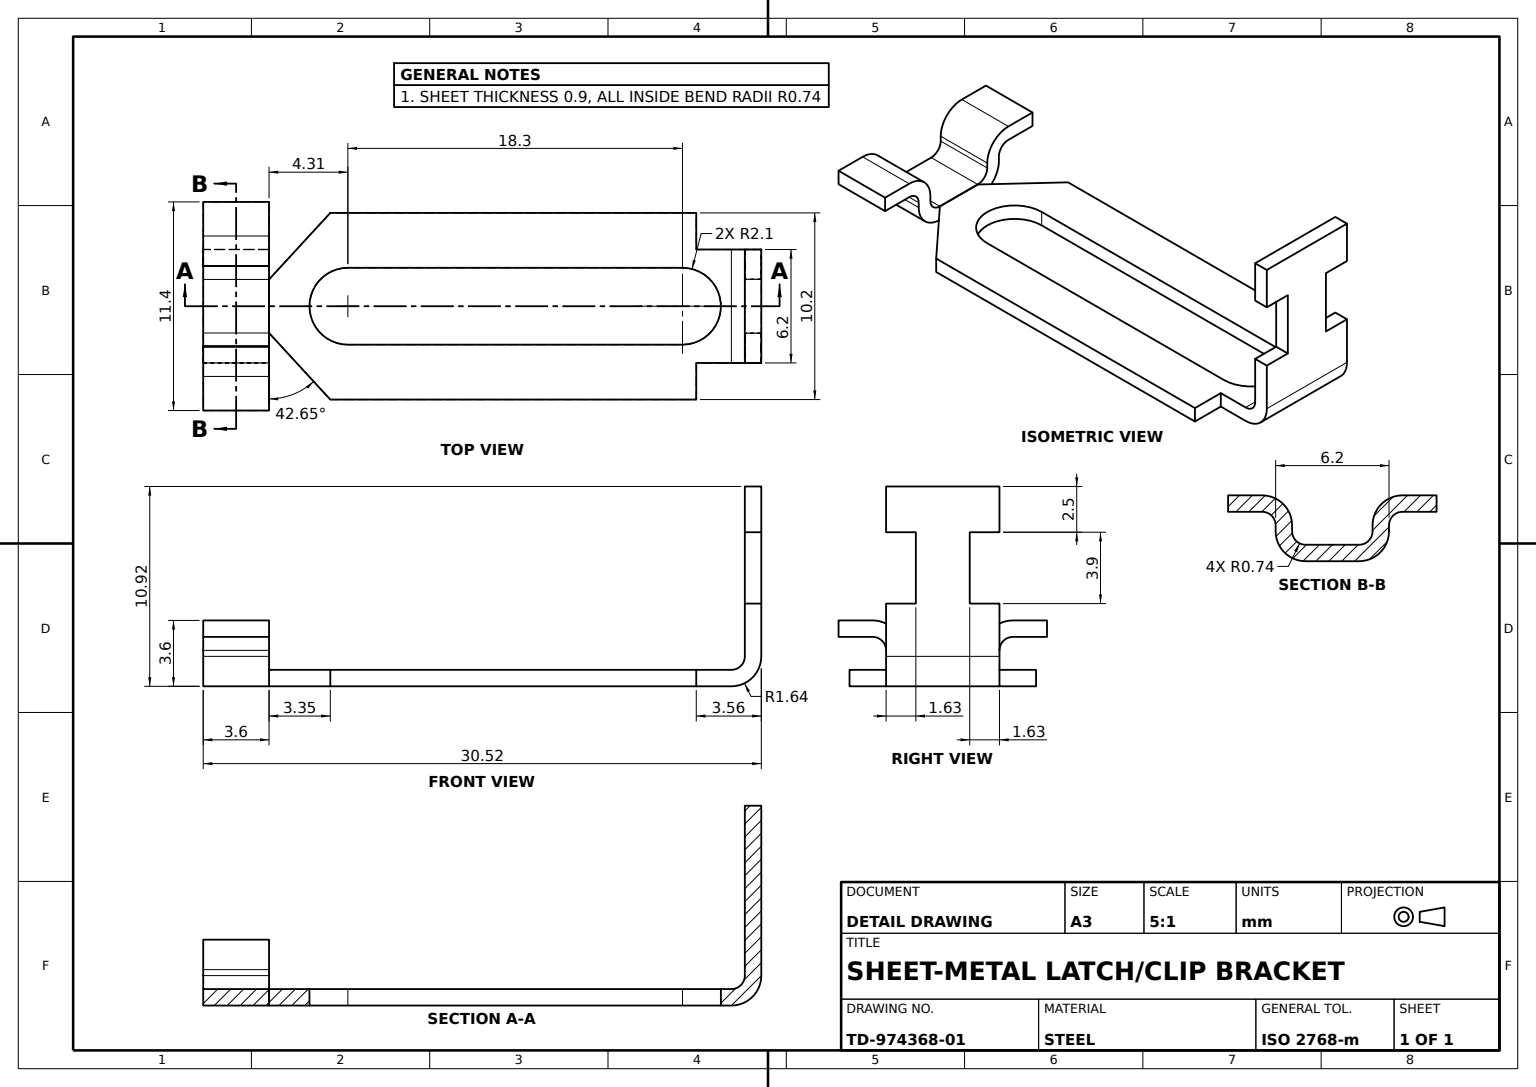
solid
v1 (1.4634,0,13.46)
v2 (1.4634,-0.9,13.46)
e1 v1 v2 LINE
v3 (5.1,-0.9,10.11)
e2 v3 v2 LINE
v4 (5.1,0,10.11)
e3 v3 v4 LINE
e4 v4 v1 LINE
face PLANE(AX(P(1.4634,-3.6,13.46),D(-0.677530464,0,-0.735494712),D(-0.735494712,0,0.677530464))) rev [e1 -e2 e3 e4]
v5 (-3.1,7.52,-12.56)
v6 (-3.1,10.02,-12.56)
e5 v5 v6 LINE
v7 (-3.1,10.02,-13.46)
e6 v7 v6 LINE
v8 (-3.1,7.52,-13.46)
e7 v7 v8 LINE
e8 v8 v5 LINE
face PLANE(AX(P(-3.1,7.958486,-9.86),D(1,0,0),D(0,1,0))) rev [e5 -e6 e7 e8]
v9 (-5.1,0,-9.9034)
v10 (-3.1,0,-9.9034)
e9 v9 v10 LINE
v11 (-3.1,-0.9,-9.9034)
e10 v11 v10 LINE
v12 (-5.1,-0.9,-9.9034)
e11 v12 v11 LINE
e12 v12 v9 LINE
face PLANE(AX(P(-5.1,-3.6,-9.9034),D(0,0,1),D(1,0,0))) rev [e9 -e10 -e11 e12]
v13 (0,0,11.25)
v14 (2.1,0,9.15)
e13 v13 v14 CIRCLE(AX(P(0,0,9.15),D(0,1,0),D(0,0,1)),2.1)
v15 (2.1,-0.9,9.15)
e14 v15 v14 LINE
v16 (0,-0.9,11.25)
e15 v16 v15 CIRCLE(AX(P(0,-0.9,9.15),D(0,1,0),D(0,0,1)),2.1)
e16 v16 v13 LINE
face CYL(AX(P(0,-3.6,9.15),D(0,1,0),D(0,0,1)),2.1) rev [e13 -e14 -e15 e16]
v17 (-3.1,3.62,-12.56)
v18 (-3.1,3.62,-13.46)
e17 v17 v18 LINE
v19 (-1.473197,3.62,-12.56)
e18 v17 v19 LINE
v20 (-1.473197,3.62,-13.46)
e19 v20 v19 LINE
e20 v18 v20 LINE
face PLANE(AX(P(-3.1,3.62,-16.16),D(0,-1,0),D(0,0,-1))) rev [-e17 e18 -e19 -e20]
v21 (3.1,10.02,-12.56)
v22 (3.1,7.52,-12.56)
e21 v21 v22 LINE
e22 v6 v21 LINE
v23 (-1.473197,7.52,-12.56)
e23 v23 v5 LINE
e24 v19 v23 LINE
v24 (-3.1,0.7366,-12.56)
e25 v24 v17 LINE
v25 (3.1,0.7366,-12.56)
e26 v25 v24 LINE
v26 (3.1,3.62,-12.56)
e27 v26 v25 LINE
v27 (1.473197,3.62,-12.56)
e28 v27 v26 LINE
v28 (1.473197,7.52,-12.56)
e29 v28 v27 LINE
e30 v22 v28 LINE
face PLANE(AX(P(0,0,-12.56),D(0,0,1),D(0,-1,0))) [-e21 -e22 -e5 -e23 -e24 -e18 -e25 -e26 -e27 -e28 -e29 -e30]
v29 (-3.1,-0.9,-11.8234)
v30 (3.1,-0.9,-11.8234)
e31 v29 v30 LINE
v31 (-3.1,0.7366,-13.46)
e32 v31 v29 CIRCLE(AX(P(-3.1,0.7366,-11.8234),D(-1,0,0),D(0,0,-1)),1.6366)
v32 (3.1,0.7366,-13.46)
e33 v31 v32 LINE
e34 v30 v32 CIRCLE(AX(P(3.1,0.7366,-11.8234),D(1,0,0),D(0,0,1)),1.6366)
face CYL(AX(P(-5.1,0.7366,-11.8234),D(-1,0,0),D(0,0,-1)),1.6366) [-e31 -e32 e33 -e34]
v33 (-2.1,-0.9,9.15)
v34 (-2.1,0,9.15)
e35 v33 v34 LINE
e36 v34 v13 CIRCLE(AX(P(0,0,9.15),D(0,1,0),D(0,0,1)),2.1)
e37 v33 v16 CIRCLE(AX(P(0,-0.9,9.15),D(0,1,0),D(0,0,1)),2.1)
face CYL(AX(P(0,-3.6,9.15),D(0,1,0),D(0,0,1)),2.1) rev [e35 e36 -e16 -e37]
v35 (-3.1,0,-11.8234)
e38 v10 v35 LINE
v36 (-5.1,0,10.11)
e39 v9 v36 LINE
v37 (-1.4634,0,13.46)
e40 v37 v36 LINE
e41 v37 v1 LINE
v38 (5.1,0,-9.9034)
e42 v4 v38 LINE
v39 (3.1,0,-9.9034)
e43 v39 v38 LINE
v40 (3.1,0,-11.8234)
e44 v40 v39 LINE
e45 v35 v40 LINE
v41 (-2.1,0,-9.15)
e46 v41 v34 LINE
v42 (2.1,0,-9.15)
e47 v42 v41 CIRCLE(AX(P(0,0,-9.15),D(0,1,0),D(0,0,1)),2.1)
e48 v14 v42 LINE
face PLANE(AX(P(0,0,0),D(0,1,0),D(0,0,1))) [-e38 -e9 e39 -e40 e41 -e4 e42 -e43 -e44 -e45] [-e36 -e46 -e47 -e48 -e13]
v43 (-1.473197,7.52,-13.46)
e49 v43 v23 LINE
e50 v20 v43 LINE
face PLANE(AX(P(-1.473197,7.52,-16.16),D(1,0,0),D(0,1,0))) rev [e19 e24 -e49 -e50]
v44 (2.1,-0.9,-9.15)
e51 v15 v44 LINE
v45 (-2.1,-0.9,-9.15)
e52 v44 v45 CIRCLE(AX(P(0,-0.9,-9.15),D(0,1,0),D(0,0,1)),2.1)
e53 v45 v33 LINE
e54 v11 v29 LINE
v46 (3.1,-0.9,-9.9034)
e55 v30 v46 LINE
v47 (5.1,-0.9,-9.9034)
e56 v46 v47 LINE
e57 v3 v47 LINE
v48 (-1.4634,-0.9,13.46)
e58 v48 v2 LINE
v49 (-5.1,-0.9,10.11)
e59 v48 v49 LINE
e60 v12 v49 LINE
face PLANE(AX(P(0,-0.9,0),D(0,1,0),D(0,0,1))) rev [e51 e52 e53 e37 e15] [e54 e31 e55 e56 -e57 e2 -e58 e59 -e60 e11]
e61 v48 v37 LINE
face PLANE(AX(P(-5.1,-0.9,13.46),D(0,0,1),D(1,0,0))) [-e61 e58 -e1 -e41]
v50 (3.1,7.52,-13.46)
e62 v22 v50 LINE
v51 (1.473197,7.52,-13.46)
e63 v51 v28 LINE
e64 v50 v51 LINE
face PLANE(AX(P(3.1,7.52,-16.16),D(0,1,0),D(-1,0,0))) rev [-e62 e30 -e63 -e64]
v52 (3.1,10.02,-13.46)
e65 v52 v21 LINE
e66 v7 v52 LINE
face PLANE(AX(P(5.1,10.02,-13.46),D(0,-1,0),D(0,0,-1))) rev [e6 e22 -e65 -e66]
e67 v44 v42 LINE
e68 v45 v41 LINE
face CYL(AX(P(0,-3.6,-9.15),D(0,1,0),D(0,0,1)),2.1) rev [e67 e47 -e68 -e52]
e69 v47 v38 LINE
face PLANE(AX(P(5.1,-0.9,-13.46),D(1,0,0),D(0,0,-1))) [-e42 -e3 e57 e69]
e70 v49 v36 LINE
face PLANE(AX(P(-1.4634,-3.6,13.46),D(0.677530464,0,-0.735494712),D(-0.735494712,0,-0.677530464))) rev [-e70 -e59 e61 e40]
e71 v46 v39 LINE
face PLANE(AX(P(5.1,-3.6,-9.9034),D(0,0,1),D(1,0,0))) rev [e43 -e69 -e56 e71]
face PLANE(AX(P(2.1,-3.6,9.15),D(1,0,0),D(0,0,-1))) rev [-e67 -e51 e14 e48]
face PLANE(AX(P(-2.1,-3.6,9.15),D(-1,0,0),D(0,0,1))) rev [e46 -e35 -e53 e68]
e72 v50 v52 LINE
v53 (1.473197,3.62,-13.46)
e73 v51 v53 LINE
v54 (3.1,3.62,-13.46)
e74 v53 v54 LINE
e75 v32 v54 LINE
e76 v18 v31 LINE
e77 v43 v8 LINE
face PLANE(AX(P(0,0,-13.46),D(0,0,1),D(0,-1,0))) rev [-e72 e64 e73 e74 -e75 -e33 -e76 e20 e50 e77 -e7 e66]
face PLANE(AX(P(-3.1,7.52,-16.16),D(0,1,0),D(0,0,1))) rev [e49 e23 -e8 -e77]
e78 v54 v26 LINE
e79 v53 v27 LINE
face PLANE(AX(P(3.1,3.62,-16.16),D(0,-1,0),D(0,0,-1))) rev [e28 -e78 -e74 e79]
e80 v40 v25 CIRCLE(AX(P(3.1,0.7366,-11.8234),D(1,0,0),D(0,0,1)),0.7366)
e81 v24 v35 CIRCLE(AX(P(-3.1,0.7366,-11.8234),D(-1,0,0),D(0,0,-1)),0.7366)
face CYL(AX(P(-5.1,0.7366,-11.8234),D(-1,0,0),D(0,0,-1)),0.7366) rev [e45 e80 e26 e81]
face PLANE(AX(P(-3.1,-3.6,-11.8234),D(1,0,0),D(0,0,-1))) rev [e38 -e81 e25 e17 e76 e32 -e54 e10]
face PLANE(AX(P(3.1,7.958486,-9.86),D(-1,0,0),D(0,-1,0))) rev [e62 e72 e65 e21]
face PLANE(AX(P(1.473197,7.52,-16.16),D(-1,0,0),D(0,-1,0))) rev [e63 e29 -e79 -e73]
face PLANE(AX(P(-5.1,-0.9,-13.46),D(-1,0,0),D(0,0,1))) [e70 -e39 -e12 e60]
face PLANE(AX(P(3.1,-3.6,-11.8234),D(-1,0,0),D(0,0,1))) rev [e78 e27 -e80 e44 -e71 -e55 e34 e75]
solid
v55 (-2.2,0.7366,17.06)
v56 (-3.1,0.7366,17.06)
e82 v55 v56 LINE
v57 (-1.4634,-0.9,17.06)
e83 v56 v57 CIRCLE(AX(P(-1.4634,0.7366,17.06),D(0,0,1),D(1,0,0)),1.6366)
v58 (-1.4634,0,17.06)
e84 v58 v57 LINE
e85 v55 v58 CIRCLE(AX(P(-1.4634,0.7366,17.06),D(0,0,1),D(1,0,0)),0.7366)
face PLANE(AX(P(-1.4634,0.7366,17.06),D(0,0,-1),D(-1,0,0))) rev [e82 e83 -e84 -e85]
v59 (3.8366,2.7,17.06)
v60 (2.2,1.0634,17.06)
e86 v59 v60 CIRCLE(AX(P(3.8366,1.0634,17.06),D(0,0,1),D(0,-1,0)),1.6366)
v61 (3.1,1.0634,17.06)
e87 v61 v60 LINE
v62 (3.8366,1.8,17.06)
e88 v62 v61 CIRCLE(AX(P(3.8366,1.0634,17.06),D(0,0,1),D(0,-1,0)),0.7366)
e89 v62 v59 LINE
face PLANE(AX(P(3.8366,1.0634,17.06),D(0,0,-1),D(0,1,0))) rev [e86 -e87 -e88 e89]
v63 (1.4634,-0.9,17.06)
e90 v57 v63 LINE
v64 (-1.4634,-0.9,13.46)
e91 v57 v64 LINE
v65 (1.4634,-0.9,13.46)
e92 v64 v65 LINE
e93 v65 v63 LINE
face PLANE(AX(P(-3.1,-0.9,17.06),D(0,1,0),D(0,0,1))) rev [-e90 e91 e92 e93]
v66 (2.2,0.7366,13.46)
v67 (3.1,0.7366,13.46)
e94 v66 v67 LINE
e95 v67 v65 CIRCLE(AX(P(1.4634,0.7366,13.46),D(0,0,-1),D(-1,0,0)),1.6366)
v68 (1.4634,0,13.46)
e96 v68 v65 LINE
e97 v66 v68 CIRCLE(AX(P(1.4634,0.7366,13.46),D(0,0,-1),D(-1,0,0)),0.7366)
face PLANE(AX(P(1.4634,0.7366,13.46),D(0,0,1),D(1,0,0))) rev [e94 e95 -e96 -e97]
v69 (2.2,0.7366,17.06)
e98 v69 v66 LINE
e99 v60 v69 LINE
v70 (2.2,1.0634,13.46)
e100 v60 v70 LINE
e101 v66 v70 LINE
face PLANE(AX(P(2.2,0,0),D(-1,0,0),D(0,-1,0))) [-e98 -e99 e100 -e101]
v71 (3.1,1.0634,13.46)
e102 v61 v71 LINE
v72 (3.8366,1.8,13.46)
e103 v71 v72 CIRCLE(AX(P(3.8366,1.0634,13.46),D(0,0,-1),D(0,-1,0)),0.7366)
e104 v72 v62 LINE
face CYL(AX(P(3.8366,1.0634,17.06),D(0,0,1),D(0,1,0)),0.7366) rev [e102 e103 e104 e88]
v73 (-3.8366,1.8,13.46)
v74 (-3.1,1.0634,13.46)
e105 v73 v74 CIRCLE(AX(P(-3.8366,1.0634,13.46),D(0,0,-1),D(0,1,0)),0.7366)
v75 (-3.1,1.0634,17.06)
e106 v74 v75 LINE
v76 (-3.8366,1.8,17.06)
e107 v75 v76 CIRCLE(AX(P(-3.8366,1.0634,17.06),D(0,0,1),D(0,1,0)),0.7366)
e108 v76 v73 LINE
face CYL(AX(P(-3.8366,1.0634,13.46),D(0,0,-1),D(0,1,0)),0.7366) rev [e105 e106 e107 e108]
v77 (-3.1,0.7366,13.46)
e109 v64 v77 CIRCLE(AX(P(-1.4634,0.7366,13.46),D(0,0,-1),D(1,0,0)),1.6366)
v78 (-2.2,0.7366,13.46)
e110 v78 v77 LINE
v79 (-1.4634,0,13.46)
e111 v79 v78 CIRCLE(AX(P(-1.4634,0.7366,13.46),D(0,0,-1),D(1,0,0)),0.7366)
e112 v79 v64 LINE
face PLANE(AX(P(-1.4634,0.7366,13.46),D(0,0,-1),D(-1,0,0))) [e109 -e110 -e111 e112]
e113 v71 v70 LINE
e114 v67 v71 LINE
face PLANE(AX(P(3.1,2.7,13.46),D(0,0,1),D(1,0,0))) rev [e101 -e113 -e114 -e94]
v80 (3.8366,2.7,13.46)
e115 v70 v80 CIRCLE(AX(P(3.8366,1.0634,13.46),D(0,0,-1),D(0,-1,0)),1.6366)
e116 v72 v80 LINE
face PLANE(AX(P(3.8366,1.0634,13.46),D(0,0,-1),D(0,1,0))) [e115 -e116 -e103 e113]
e117 v78 v55 LINE
e118 v58 v79 LINE
face CYL(AX(P(-1.4634,0.7366,17.06),D(0,0,1),D(-1,0,0)),0.7366) rev [e111 e117 e85 e118]
v81 (-5.7,2.7,13.46)
v82 (-5.7,1.8,13.46)
e119 v81 v82 LINE
v83 (-5.7,1.8,17.06)
e120 v82 v83 LINE
v84 (-5.7,2.7,17.06)
e121 v84 v83 LINE
e122 v81 v84 LINE
face PLANE(AX(P(-5.7,2.7,17.06),D(1,0,0),D(0,1,0))) rev [e119 e120 -e121 -e122]
v85 (-2.2,1.0634,17.06)
v86 (-3.8366,2.7,17.06)
e123 v85 v86 CIRCLE(AX(P(-3.8366,1.0634,17.06),D(0,0,1),D(0,1,0)),1.6366)
e124 v76 v86 LINE
e125 v75 v85 LINE
face PLANE(AX(P(-3.8366,1.0634,17.06),D(0,0,1),D(0,-1,0))) [e123 -e124 -e107 e125]
v87 (1.4634,0,17.06)
e126 v87 v69 CIRCLE(AX(P(1.4634,0.7366,17.06),D(0,0,1),D(-1,0,0)),0.7366)
e127 v68 v87 LINE
face CYL(AX(P(1.4634,0.7366,13.46),D(0,0,-1),D(1,0,0)),0.7366) rev [e126 e98 e97 e127]
v88 (-3.8366,2.7,13.46)
e128 v88 v81 LINE
e129 v73 v88 LINE
e130 v73 v82 LINE
face PLANE(AX(P(-5.7,2.7,13.46),D(0,0,1),D(1,0,0))) rev [-e119 -e128 -e129 e130]
e131 v83 v76 LINE
face PLANE(AX(P(0,1.8,0),D(0,-1,0),D(0,0,-1))) [-e108 -e131 -e120 -e130]
e132 v84 v86 LINE
e133 v88 v86 LINE
face PLANE(AX(P(0,2.7,0),D(0,-1,0),D(0,0,-1))) rev [e132 -e133 e128 e122]
v89 (5.7,2.7,17.06)
v90 (5.7,1.8,17.06)
e134 v89 v90 LINE
e135 v59 v89 LINE
e136 v62 v90 LINE
face PLANE(AX(P(5.7,2.7,17.06),D(0,0,-1),D(-1,0,0))) rev [-e134 -e135 -e89 e136]
face PLANE(AX(P(-3.1,2.7,17.06),D(0,0,-1),D(-1,0,0))) rev [e131 e124 -e132 e121]
e137 v87 v63 LINE
v91 (3.1,0.7366,17.06)
e138 v63 v91 CIRCLE(AX(P(1.4634,0.7366,17.06),D(0,0,1),D(-1,0,0)),1.6366)
e139 v69 v91 LINE
face PLANE(AX(P(1.4634,0.7366,17.06),D(0,0,1),D(1,0,0))) [e137 e138 -e139 -e126]
e140 v79 v68 LINE
face PLANE(AX(P(0,0,13.46),D(0,0,-1),D(-1,0,0))) [e96 -e92 -e112 e140]
e141 v59 v80 LINE
face CYL(AX(P(3.8366,1.0634,17.06),D(0,0,1),D(0,1,0)),1.6366) [-e115 -e100 -e86 e141]
e142 v55 v85 LINE
v92 (-2.2,1.0634,13.46)
e143 v92 v78 LINE
e144 v92 v85 LINE
face PLANE(AX(P(-2.2,0,0),D(1,0,0),D(0,1,0))) [-e142 -e117 -e143 e144]
e145 v58 v87 LINE
face PLANE(AX(P(-3.1,0,17.06),D(0,1,0),D(0,0,1))) [e145 -e127 -e140 -e118]
e146 v74 v77 LINE
e147 v74 v92 LINE
face PLANE(AX(P(-3.1,0,13.46),D(0,0,1),D(1,0,0))) rev [-e146 e147 e143 e110]
e148 v56 v77 LINE
face CYL(AX(P(-1.4634,0.7366,17.06),D(0,0,1),D(-1,0,0)),1.6366) [-e91 -e83 e148 -e109]
e149 v67 v91 LINE
face CYL(AX(P(1.4634,0.7366,13.46),D(0,0,-1),D(1,0,0)),1.6366) [-e95 e149 -e138 -e93]
v93 (5.7,1.8,13.46)
e150 v90 v93 LINE
e151 v93 v72 LINE
face PLANE(AX(P(0,1.8,0),D(0,-1,0),D(0,0,-1))) [-e150 -e136 -e104 -e151]
e152 v61 v91 LINE
face PLANE(AX(P(3.1,0,0),D(-1,0,0),D(0,-1,0))) rev [e114 -e102 e152 -e149]
v94 (5.7,2.7,13.46)
e153 v94 v93 LINE
e154 v89 v94 LINE
face PLANE(AX(P(5.7,2.7,13.46),D(-1,0,0),D(0,-1,0))) rev [e150 -e153 -e154 e134]
e155 v94 v80 LINE
face PLANE(AX(P(3.1,2.7,13.46),D(0,0,1),D(1,0,0))) rev [e116 -e155 e153 e151]
face PLANE(AX(P(3.1,0,17.06),D(0,0,-1),D(-1,0,0))) rev [e99 e139 -e152 e87]
face PLANE(AX(P(0,0,17.06),D(0,0,-1),D(-1,0,0))) rev [-e145 e84 e90 -e137]
e156 v56 v75 LINE
face PLANE(AX(P(-3.1,2.7,17.06),D(0,0,-1),D(-1,0,0))) rev [-e82 e142 -e125 -e156]
face PLANE(AX(P(0,2.7,0),D(0,-1,0),D(0,0,-1))) rev [e155 -e141 e135 e154]
e157 v88 v92 CIRCLE(AX(P(-3.8366,1.0634,13.46),D(0,0,-1),D(0,1,0)),1.6366)
face PLANE(AX(P(-3.8366,1.0634,13.46),D(0,0,1),D(0,-1,0))) rev [e129 e157 -e147 -e105]
face PLANE(AX(P(-3.1,0,0),D(1,0,0),D(0,1,0))) rev [e146 -e148 e156 -e106]
face CYL(AX(P(-3.8366,1.0634,13.46),D(0,0,-1),D(0,1,0)),1.6366) [-e144 -e157 e133 -e123]
